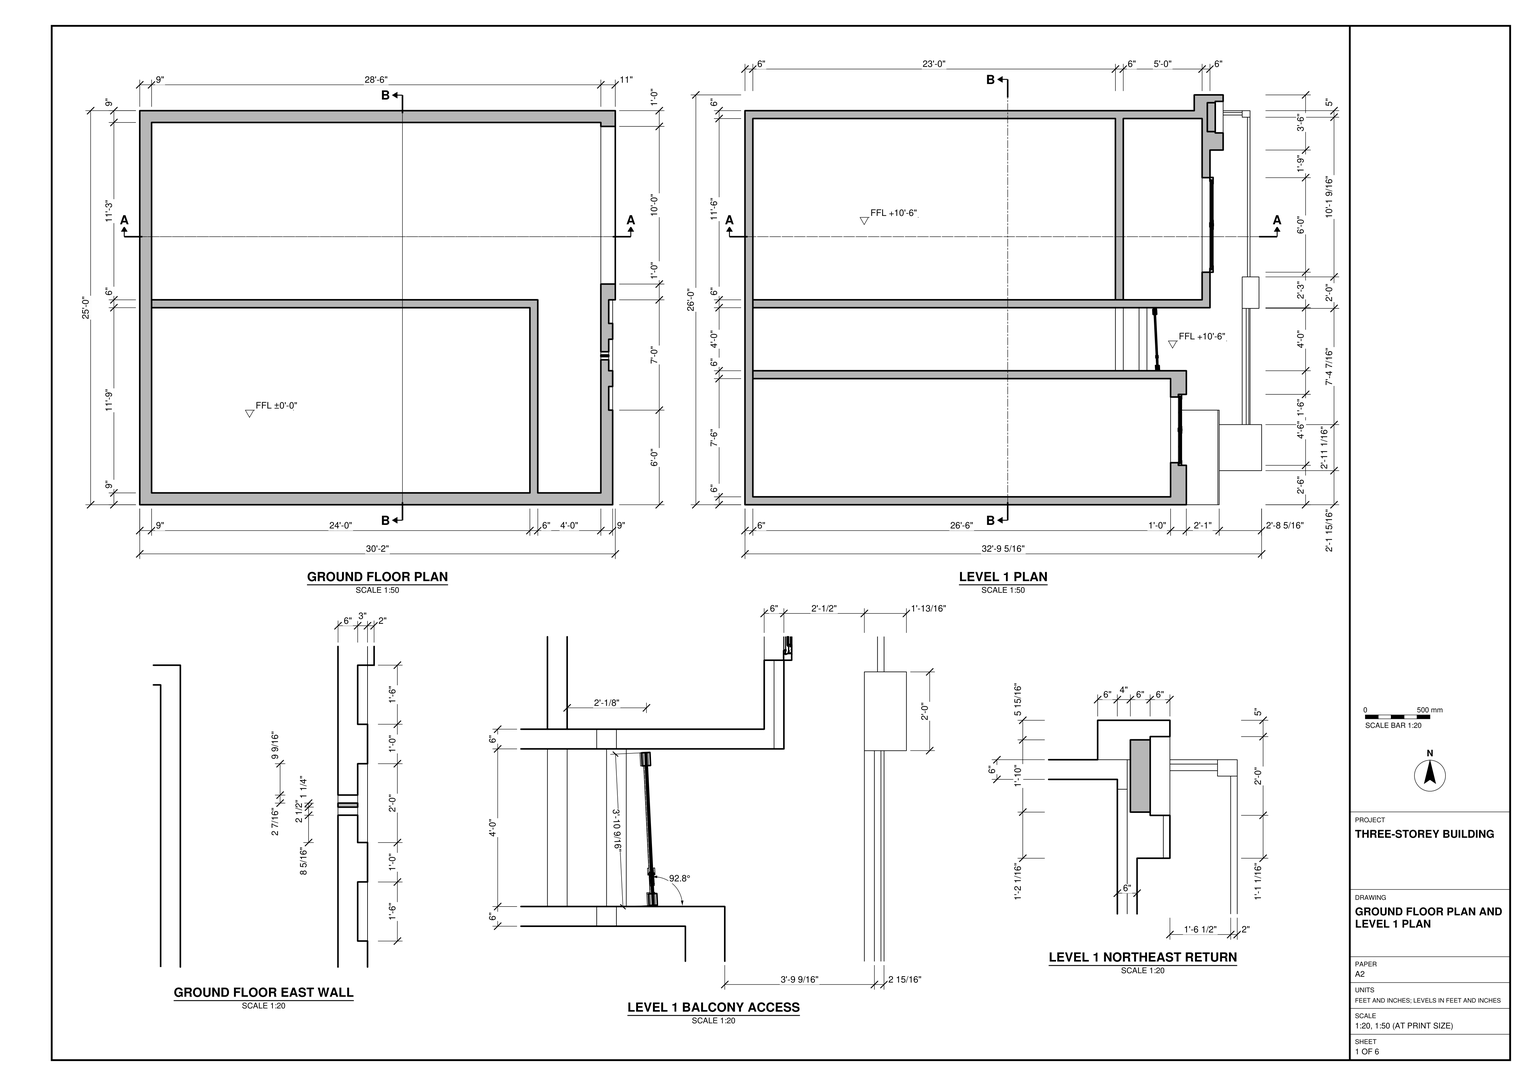
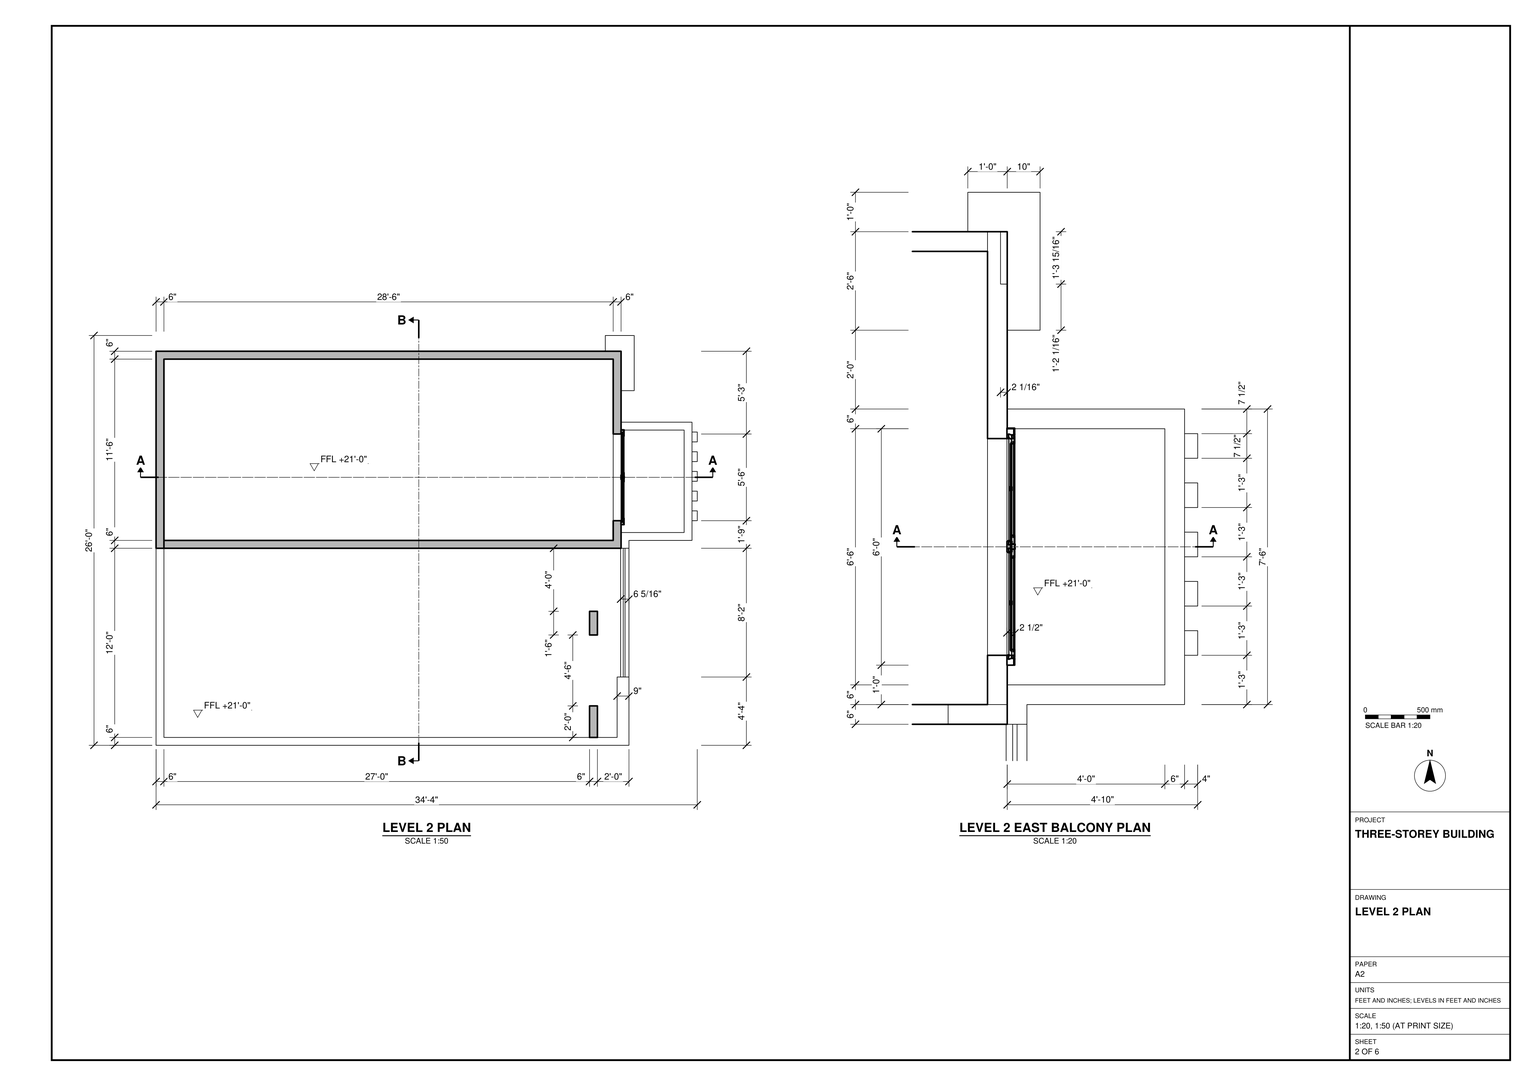
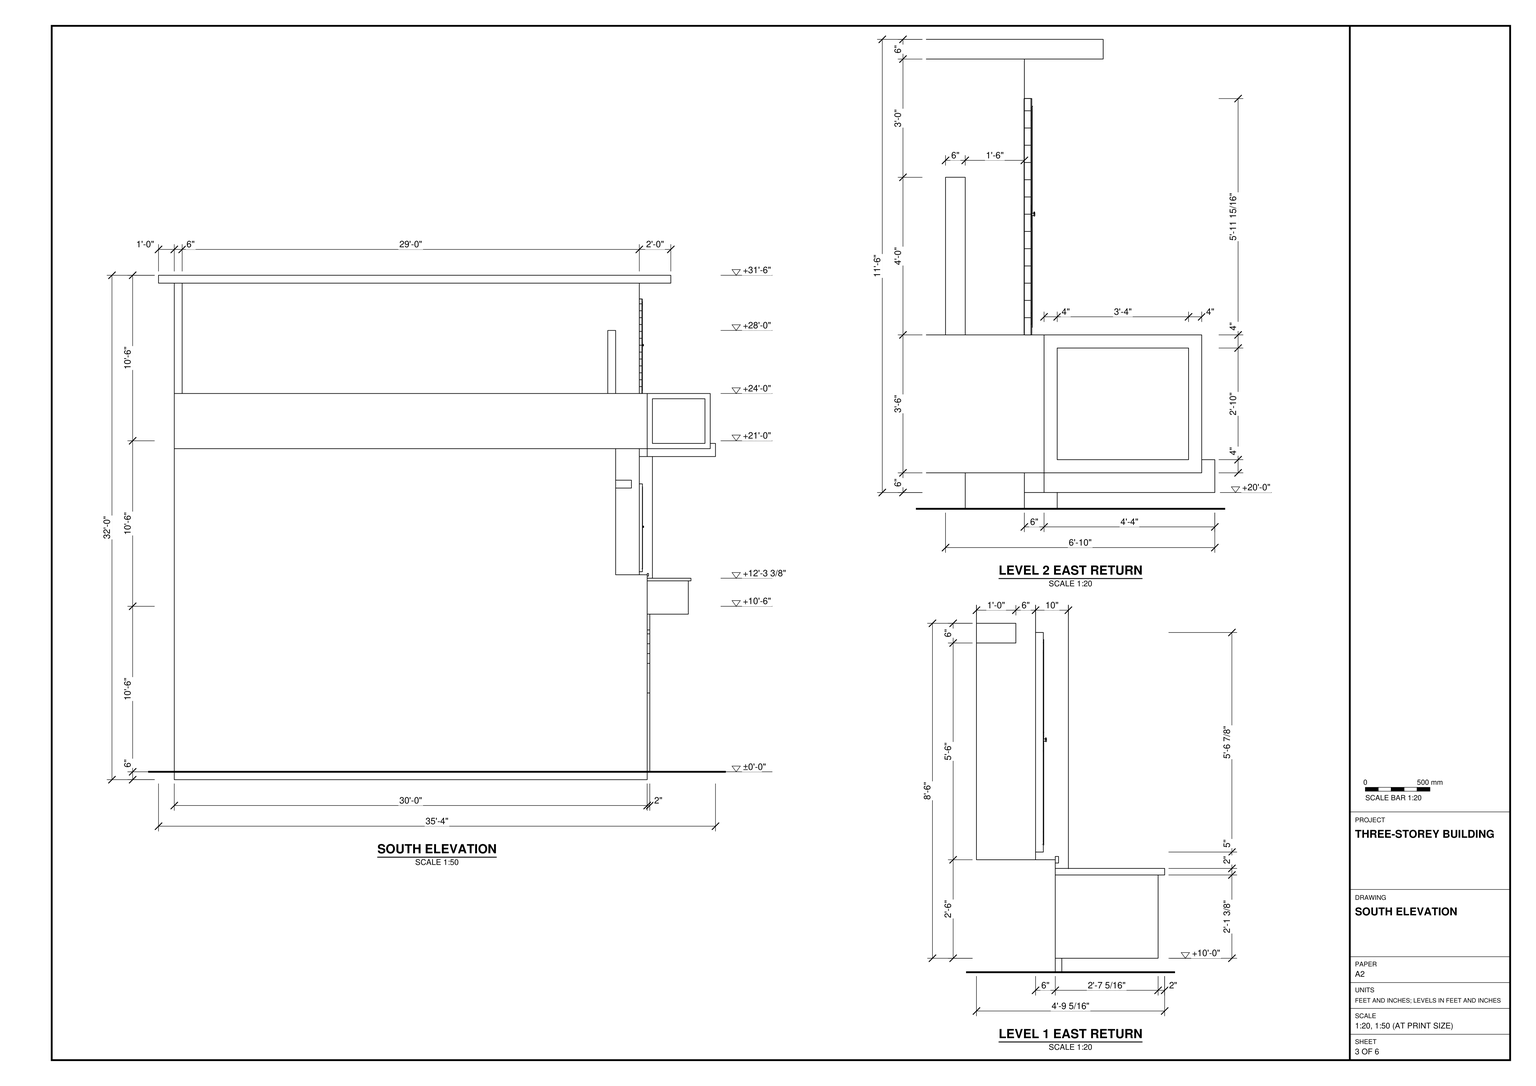
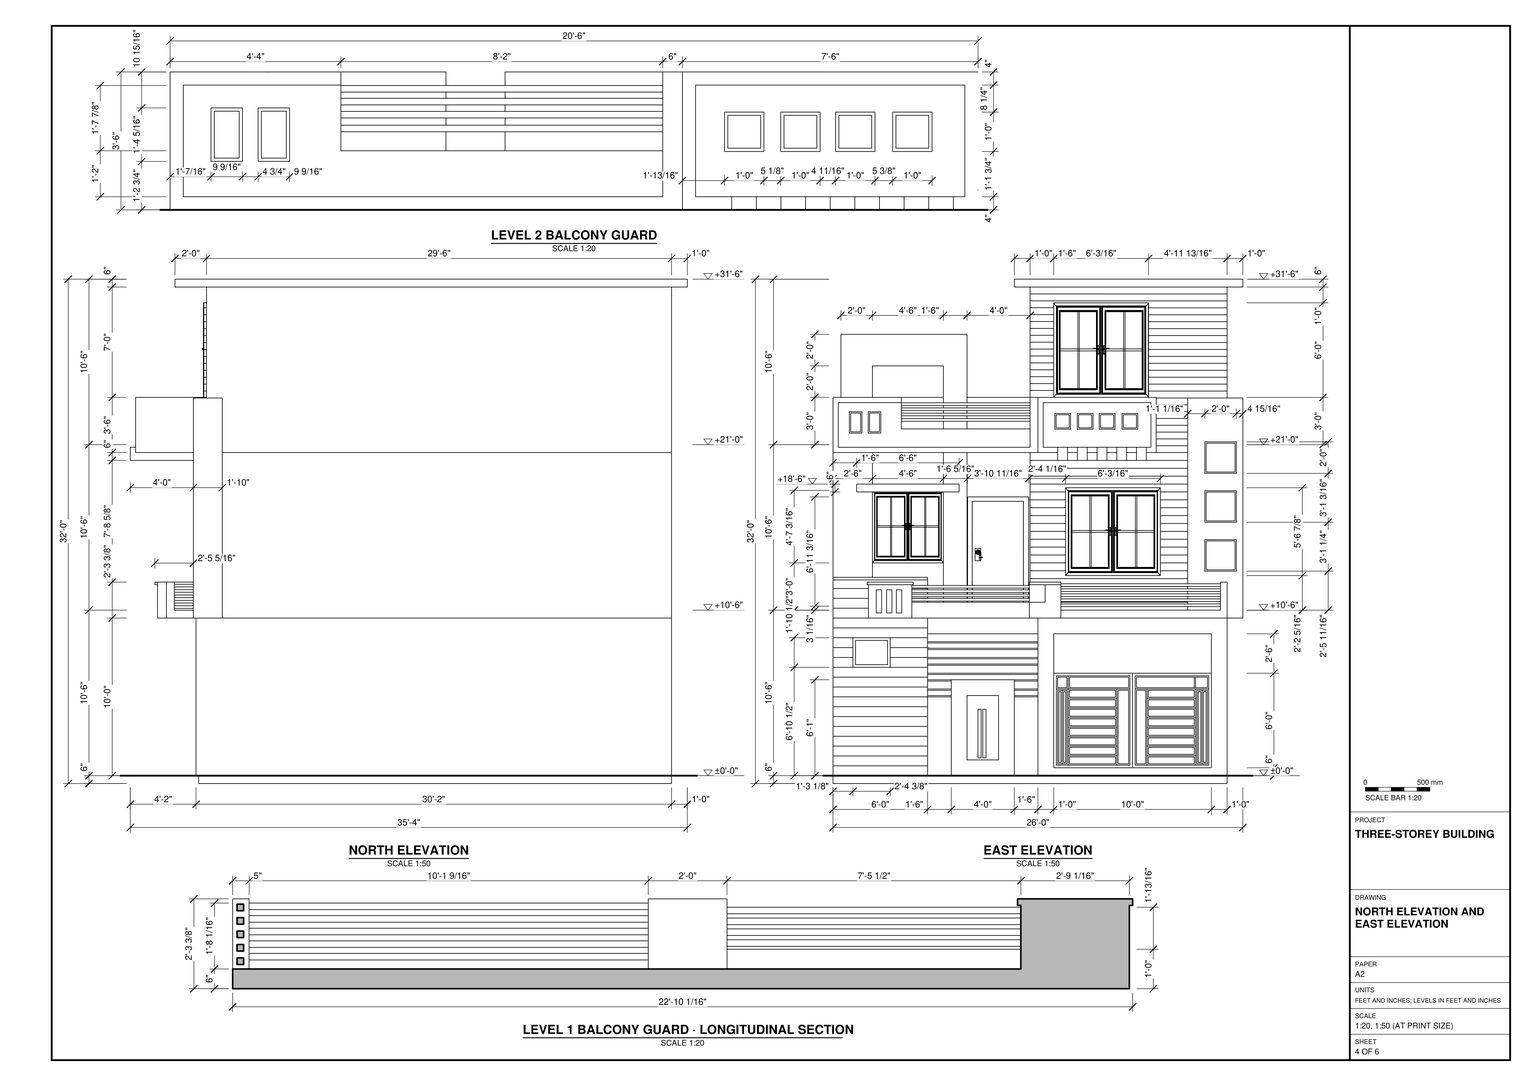
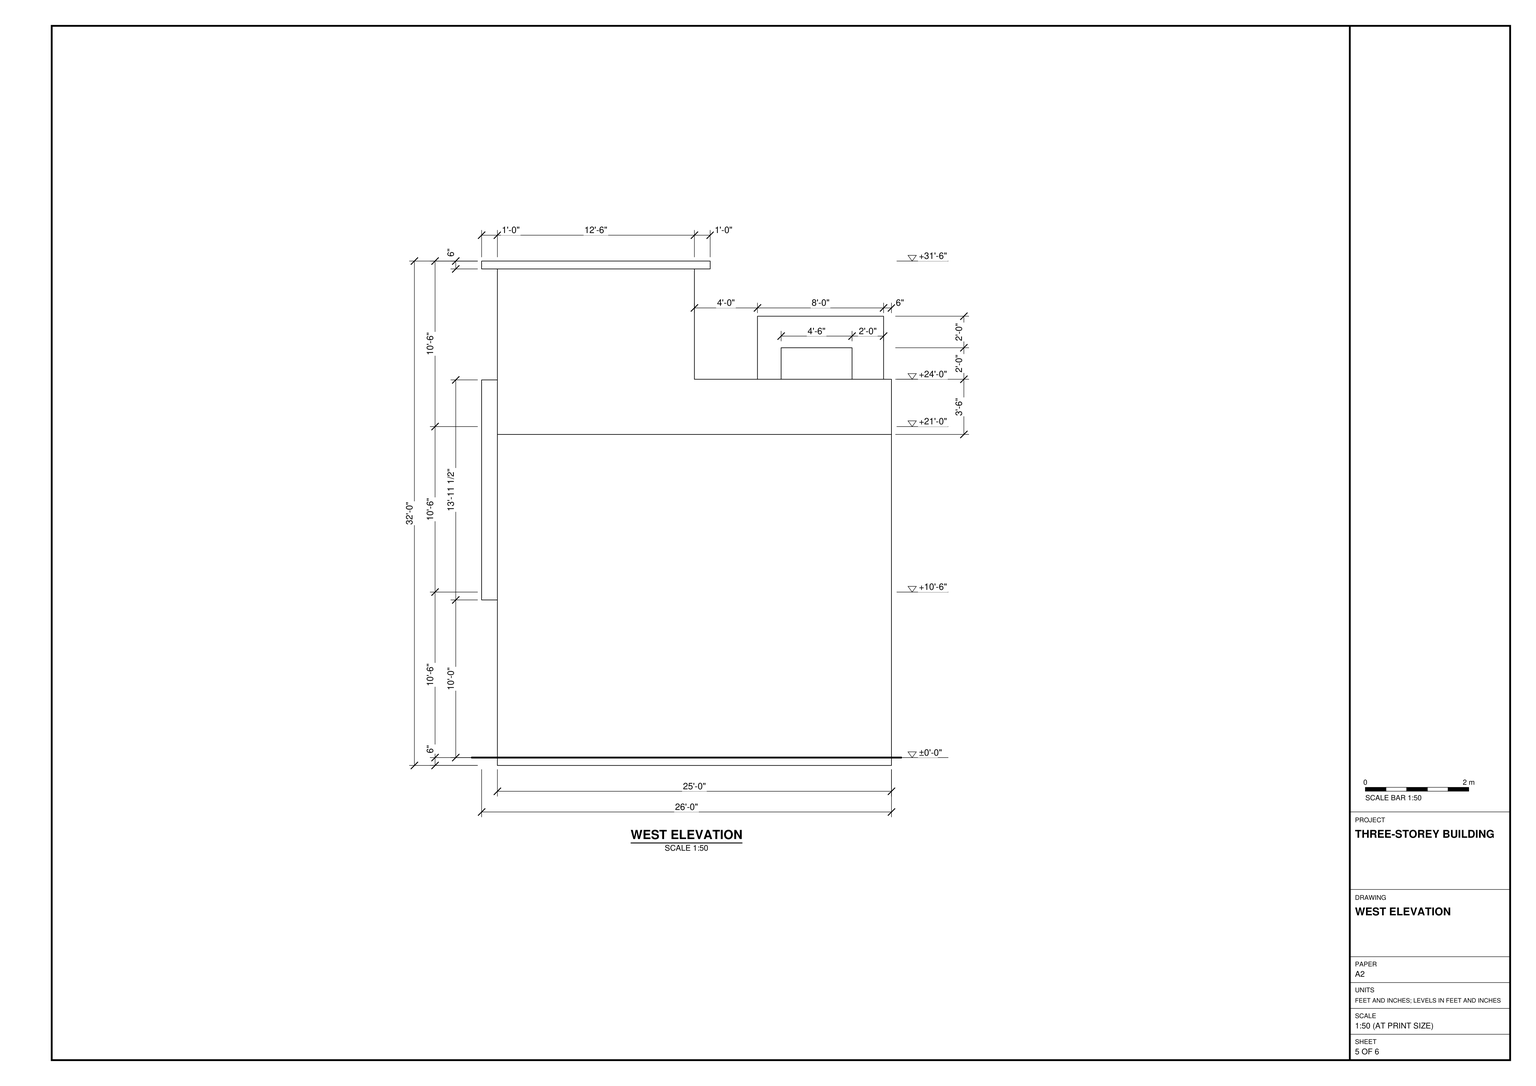
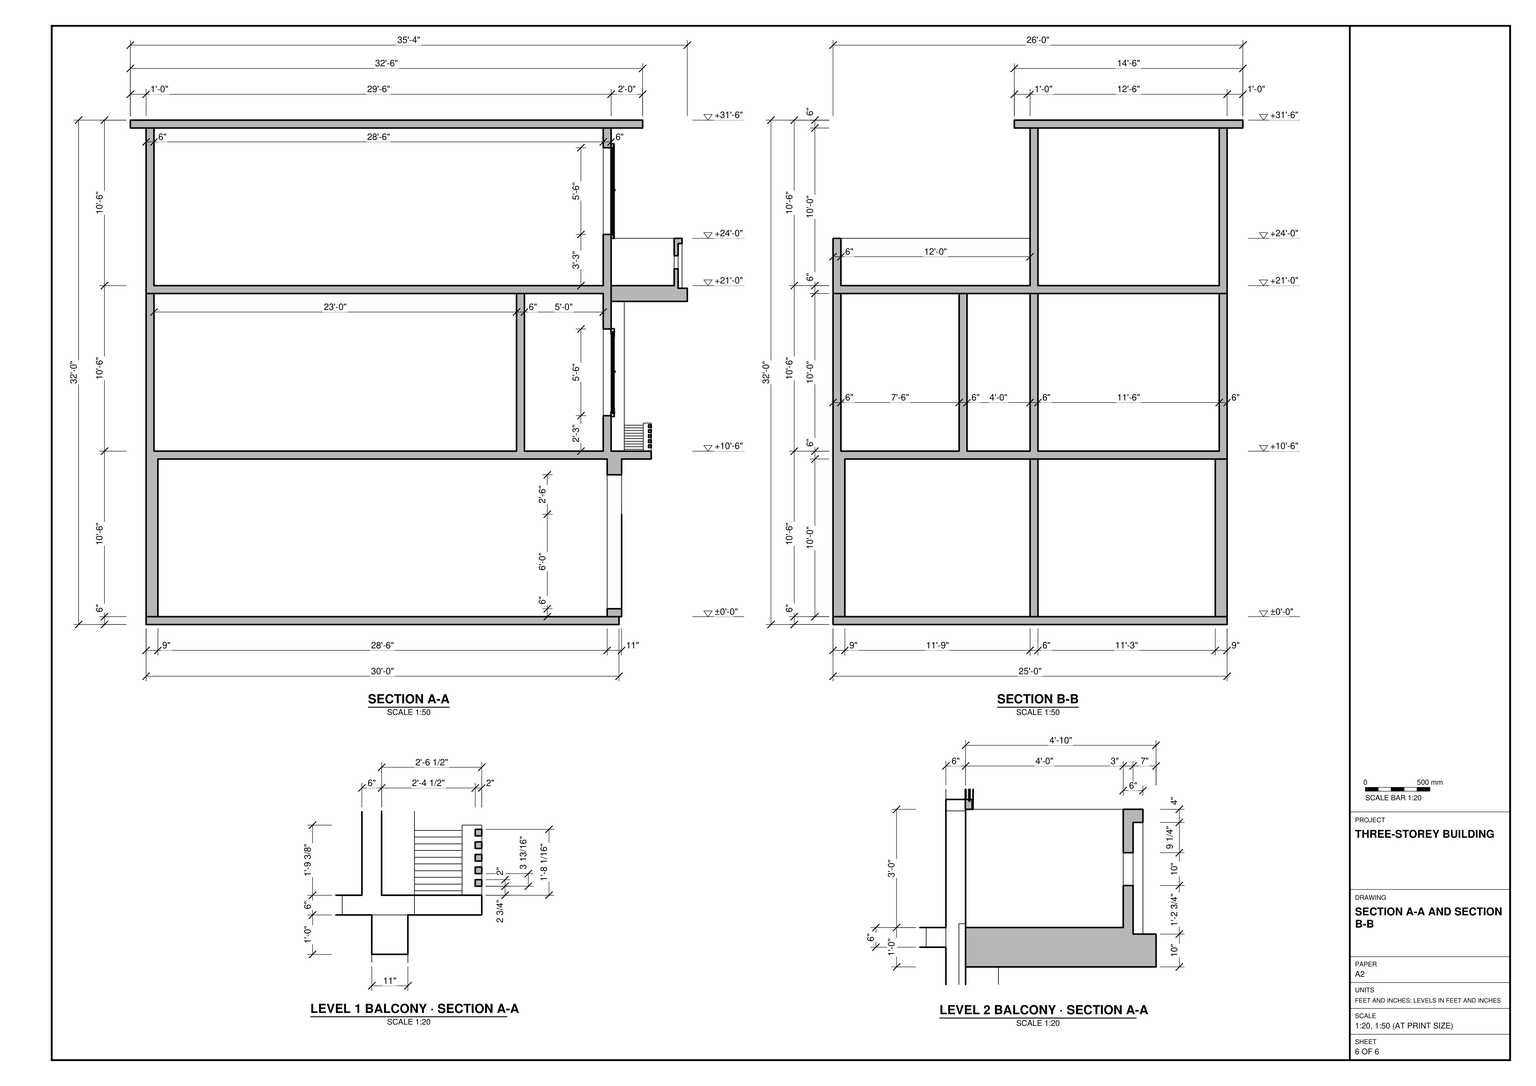
Build the three-storey building in SketchUp from task_files/diagram_01.pdf. Work in feet and inches. The overall model measures 35'-4" east to west, 26'-0" north to south and 32'-0" from the underside of the base slab to the top of the roof. Set the finished floor levels at ±0'-0", +10'-6" and +21'-0".

Follow the wall thicknesses on each plan rather than using one thickness throughout. On the ground floor, model the 9" perimeter walls where indicated and the 6" partition that turns south near the east wall. Form the east wall openings and recesses as drawn. On Level 1, divide the north room to form the narrow east bay and leave the passage between the north and south rooms leading to the balcony. On Level 2, enclose the north room and retain the terrace to its south. Use the enlarged balcony plans and return details to model the access openings, projecting slabs, balcony edges and repeated projections on the upper balcony face. Match the flat roof overhangs to the south elevation.

Include stairs, built-in joinery and main furniture only where shown. Keep walls, slabs, the roof and each furniture or joinery piece in separate groups or components, and use components for repeated parts. Any decor or loose items shown may be represented by suitable library components. Save one SketchUp model as output_files/three_storey_building_with_balconies_and_south_terrace.skp.

# SketchUp Ruby script. Lengths in inches.
U = 1.inch
M = Sketchup.active_model
def pt(a) = Geom::Point3d.new(a.map { |v| v * U })
def face(e, loops, mat)
  f = e.add_face(loops[0].map { |a| pt(a) })
  loops[1..].each { |l| e.add_face(l.map { |a| pt(a) }).erase! }
  f.material = f.back_material = mat if mat
  f
end
# faces: each face lists its corners as indices into pts; further lists are holes
def faces(e, pts, list, mat = nil) = list.each { |f| face(e, (f[0].is_a?(Array) ? f : [f]).map { |l| l.map { |i| pts[i] } }, mat) }
# xy, xz, yz: faces in a plane at the given z, y or x. An outline is a flat list of corners, or four numbers for a rectangle; further outlines are holes
def ring(l) = l.size == 4 ? [[l[0], l[1]], [l[2], l[1]], [l[2], l[3]], [l[0], l[3]]] : l.each_slice(2).to_a
def flat(e, list, mat, &to3) = list.each { |f| face(e, (f[0].is_a?(Array) ? f : [f]).map { |l| ring(l).map { |u, v| to3.(u, v) } }, mat) }
def xy(e, z, list, mat = nil) = flat(e, list, mat) { |x, y| [x, y, z] }
def xz(e, y, list, mat = nil) = flat(e, list, mat) { |x, z| [x, y, z] }
def yz(e, x, list, mat = nil) = flat(e, list, mat) { |y, z| [x, y, z] }
def lines(e, pts, list) = list.each { |a, b| e.add_line(pt(pts[a]), pt(pts[b])) }
# prism: a flat outline (further loops are holes) pulled along v
def prism(e, loops, v, mat = nil)
  f = face(e, loops, mat); d = Geom::Vector3d.new(v.map { |x| x * U })
  f.pushpull(f.normal.samedirection?(d) ? d.length : -d.length)
end
def box(e, o, s, mat = nil) = prism(e, [[o, [o[0] + s[0], o[1], o[2]], [o[0] + s[0], o[1] + s[1], o[2]], [o[0], o[1] + s[1], o[2]]]], [0, 0, s[2]], mat)
def at(x, y, z, deg = 0) = Geom::Transformation.translation(pt([x, y, z])) * Geom::Transformation.rotation(ORIGIN, Z_AXIS, deg.degrees)
def axes(o, x, y, z) = Geom::Transformation.new([*x, 0, *y, 0, *z, 0, *pt(o).to_a, 1])
def part(name) = M.definitions.add(name)
# library, detail: a bought-in or finely detailed component or shape, given as its bounding box
def library(name, o, s) = part(name).tap { |d| box(d.entities, o, s) }
def detail(e, o, s) = box(e.add_group.entities, o, s)
def put(e, d, t, mat = nil) = e.add_instance(d, t).tap { |i| i.material = mat if mat }
def group(e, t, mat = nil) = e.add_group.tap { |g| g.transformation = t; g.material = mat if mat }.entities
root = M.entities
M.materials.add("A08_Garnet_Shadow").color = [102, 0, 0]
M.materials.add("D07_Ochre_Flame").color = [153, 107, 0]
M.materials.add("Denim_03_1K").color = [93, 106, 119]
M.materials.add("Glass_Basic_01").color = [75, 19, 186]
M.materials["Glass_Basic_01"].alpha = 0.25
M.materials.add("Wood_Veneer_15_1K").color = [103, 69, 45]
c1 = library("porta+4",[0.2,-5.42,1.33],[46.55,4.72,83.21])
c2 = library("mesh-163",[-551.08,-704.17,-20.03],[1929.24,1401.85,86.96])
c3 = part("Group11\#1")
put(c3.entities,c2,at(0,0,0))
xy(root,-6,[[12,0,372,300]])
xy(root,0,[[12,0,309,9],[309,0,309,150,21,150,21,156,315,156,315,0],[315,0,372,9],[12,9,21,150],[21,9,309,150],
  [315,9,363,9,363,291,21,291,21,156,315,156],[363,9,363,291,372,291,372,156,369,156,369,138,372,138,372,90,369,90,369,72,372,72,372,9],[369,72,372,90],[369,138,372,156],[12,150,21,156],
  [12,156,21,300],[21,291,372,300]])
xy(root,0,[[372,156,374,291],[372,291,374,300]],"Wood_Veneer_15_1K")
xy(root,6,[[363,168,374,288]],"Wood_Veneer_15_1K")
xy(root,12,[[369,102,372,126]])
xy(root,13.55,[[363,110.32,369,112.77],[363,114,369,116.45]],"D07_Ochre_Flame")
xy(root,50.58,[[363,110.32,369,112.77],[363,114,369,116.45]],"D07_Ochre_Flame")
xy(root,61,[[363,72,369,90],[369,102,372,126],[363,138,369,156]])
xy(root,65,[[363,72,369,90],[363,138,369,156]])
xy(root,66,[[363,72,369,90],[363,138,369,156]])
xy(root,72,[[363,72,369,90],[363,138,369,156]])
xy(root,73,[[363,72,369,72,369,90,372,90,372,138,369,138,369,156,363,156]])
xy(root,77,[[363,72,369,90],[363,90,369,138],[363,138,369,156]])
xy(root,78,[[363,72,369,156]])
xy(root,82.5,[[372,15.15,374,43.52]])
xy(root,84,[[363,72,369,90],[363,90,369,138],[363,138,369,156]])
xy(root,84.5,[[363,17.15,374,41.52]],"Denim_03_1K")
xy(root,85,[[363,72,369,156]])
xy(root,89,[[363,72,369,90],[363,90,369,138],[363,138,369,156]])
xy(root,90,[[363,72,369,90],[363,90,369,156]])
xy(root,96,[[363,72,369,90],[363,90,369,138],[363,138,369,156]])
xy(root,97,[[363,72,369,73],[363,73,369,90],[363,90,369,156]])
xy(root,101,[[363,72,369,90],[363,90,369,138],[363,138,369,156]])
xy(root,102,[[363,72,369,90],[363,90,369,156]])
xy(root,103,[[363,17.15,374,41.52]],"Denim_03_1K")
xy(root,105,[[372,15.15,374,43.52]])
xy(root,108,[[363,72,372,156]])
xy(root,108,[[363,168,374,288]],"Wood_Veneer_15_1K")
xy(root,120,[[21,9,309,150],[315,9,363,291],[372,26.95,372,156,403.3125,156,403.3125,149.46,396.5,149.46,396.5,60,403.3125,60,403.3125,26.95],[21,150,309,156],[21,156,309,291],
  [309,156,315,291],[374,156,374,300,396.5,300,396.5,173.46,403.3125,173.46,403.3125,156],[21,291,309,300],[309,291,315,300],[315,291,363,300]])
xy(root,120,[[354,300,376,312]],"D07_Ochre_Flame")
xy(root,123.88,[[398.5,32.9,403.3125,36.99],[398.5,40.77,403.3125,44.86],[398.5,48.2,403.3125,52.29]])
xy(root,126,[[18,6,336,96],[372,60,390.5,60,390.5,173.46,396.5,173.46,396.5,295,390.5,295,390.5,300,376,300,376,270,366,270,366,150,318,150,318,102,348,102,348,84,342,84,342,72,372,72],[18,102,294,150],[294,102,300,150],[300,102,312,150],
  [312,102,318,150],[18,156,294,294],[300,156,360,294]])
xy(root,127.37,[[376,296.66,390.5,298.66]])
xy(root,128.75,[[394.5,173.46,396.5,295]])
xy(root,129.37,[[376,296.66,390.5,298.66]])
xy(root,130.75,[[394.5,173.46,396.5,295]])
xy(root,131.46,[[376,296.66,390.5,298.66]])
xy(root,132,[[390.5,60,396.5,149.46]])
xy(root,132,[[396.5,149.46,403.3125,161.46]],"D07_Ochre_Flame")
xy(root,132.58,[[394.5,173.46,396.5,295]])
xy(root,132.91,[[393.55,60,395.55,149.46]])
xy(root,133.46,[[376,296.66,390.5,298.66]])
xy(root,134.58,[[394.5,173.46,396.5,295]])
xy(root,134.91,[[393.55,60,395.55,149.46]])
xy(root,135.55,[[376,296.66,390.5,298.66]])
xy(root,136.21,[[393.55,60,395.55,149.46]])
xy(root,136.41,[[394.5,173.46,396.5,295]])
xy(root,137.55,[[376,296.66,390.5,298.66]])
xy(root,138.21,[[393.55,60,395.55,149.46]])
xy(root,138.41,[[394.5,173.46,396.5,295]])
xy(root,139.51,[[393.55,60,395.55,149.46]])
xy(root,139.64,[[376,296.66,390.5,298.66]])
xy(root,140.24,[[394.5,173.46,396.5,295]])
xy(root,141.5,[[398.5,32.9,403.3125,36.99],[398.5,40.77,403.3125,44.86],[398.5,48.2,403.3125,52.29]])
xy(root,141.51,[[393.55,60,395.55,149.46]])
xy(root,141.64,[[376,296.66,390.5,298.66]])
xy(root,142.24,[[394.5,173.46,396.5,295]])
xy(root,142.8125,[[393.55,60,395.55,149.46]])
xy(root,143.73,[[376,296.66,390.5,298.66]])
xy(root,144.08,[[394.5,173.46,396.5,295]])
xy(root,144.8125,[[393.55,60,395.55,149.46]])
xy(root,145.36,[[372,25.95,396,26.95],[396,25.95,396.5,26.95],[396.5,25.95,405.3125,26.95],[403.3125,26.95,405.3125,60],[372,60,396.5,61],
  [396.5,60,405.3125,61]])
xy(root,145.36,[[396.5,149.46,403.3125,161.46]],"D07_Ochre_Flame")
xy(root,145.73,[[376,296.66,390.5,298.66]])
xy(root,146.08,[[394.5,173.46,396.5,295]])
xy(root,147.36,[[372,25.95,405.3125,61],[390.5,149.46,403.3125,173.46],[390.5,295,396.5,300]])
xy(root,149,[[372,0,373,9],[372,9,373,72]])
xy(root,150,[[348,0,372,0,372,72,342,72,342,30,348,30]])
xy(root,151,[[372,0,373,72]])
xy(root,153,[[360,177,366,249]])
xy(root,155.71,[[370,283.04,376,307.04]],"D07_Ochre_Flame")
xy(root,156.71,[[363.96,284.04,370,306.04]])
xy(root,164,[[336,32,342,82]])
xy(root,178.71,[[363.96,284.04,370,306.04]])
xy(root,179.71,[[370,283.04,376,307.04]],"D07_Ochre_Flame")
xy(root,192.9375,[[370,283.04,376,307.04]],"D07_Ochre_Flame")
xy(root,193.9375,[[363.96,284.04,370,306.04]])
xy(root,210,[[312,102,318,150]])
xy(root,214,[[336,32,342,82]])
xy(root,215.9375,[[363.96,284.04,370,306.04]])
xy(root,216,[[348,18,348,30,342,30,342,84,348,84,348,96,360,96,360,18]])
xy(root,216.9375,[[370,283.04,376,307.04]],"D07_Ochre_Flame")
xy(root,219,[[360,177,366,249]])
xy(root,222,[[348,18,360,18,360,96,348,96,348,84,342,84,342,30,348,30]])
xy(root,230.15,[[370,283.04,376,307.04]],"D07_Ochre_Flame")
xy(root,231.15,[[363.96,284.04,370,306.04]])
xy(root,240,[[366,171,424,178.5],[366,186,424,193.5],[366,201,424,208.5],[366,216,424,223.5],[366,231,424,238.5]],"A08_Garnet_Shadow")
xy(root,246,[[12,0,18,294],[18,0,294,6],[294,0,300,6],[300,0,348,6],[348,0,348,30,342,30,342,84,348,84,348,102,318,102,318,150,366,150,366,171,420,171,420,156,372,156,372,0],
  [18,6,336,96],[336,6,348,6,348,30,342,30,342,84,348,84,348,96,336,96],[18,96,294,102],[294,96,300,102],[300,96,348,96,348,102,318,102,318,150,312,150,312,102,300,102],
  [18,102,294,150],[294,102,300,150],[300,102,312,150],[18,150,294,156],[294,150,300,156],
  [300,150,318,156],[318,150,348,156],[348,150,366,156],[18,156,294,294],[294,156,300,300],
  [300,156,360,294],[366,178.5,420,186],[366,193.5,420,201],[366,208.5,420,216],[366,223.5,420,231],
  [366,238.5,420,246],[12,294,294,300],[300,294,360,300]])
xy(root,250,[[369,4,372,6],[369,6,372,30],[369,30,372,84],[369,84,372,150],[376,156,416,159],
  [417,160,420,171],[417,178.5,420,186],[417,193.5,420,201],[417,208.5,420,216],[417,223.5,420,231],
  [417,238.5,420,242]])
xy(root,250,[[417,171,424,178.5],[417,186,424,193.5],[417,201,424,208.5],[417,216,424,223.5],[417,231,424,238.5]],"A08_Garnet_Shadow")
xy(root,252,[[18,6,342,6,342,30,348,30,348,6,363,6,363,52,366,52,366,150,18,150],[342,6,348,30],[18,156,360,294],[366,162,414,240]])
xy(root,253.15,[[363.96,284.04,370,306.04]])
xy(root,254.15,[[370,283.04,376,307.04]],"D07_Ochre_Flame")
xy(root,260.76,[[369,12.45,370,22.03],[369,26.8,370,36.38]])
xy(root,261.76,[[369,13.45,370,21.03],[369,27.8,370,35.38]])
xy(root,264,[[366,52,369,150]])
xy(root,264.78,[[414,169.82,417,179.82],[414,186.93,417,196.93],[414,203.64,417,213.64],[414,221.01,417,231.01]])
xy(root,269.79,[[365.66,52,367.66,150]])
xy(root,271.79,[[365.66,52,367.66,150]])
xy(root,273.99,[[365.66,52,367.66,150]])
xy(root,274.78,[[414,169.82,417,179.82],[414,186.93,417,196.93],[414,203.64,417,213.64],[414,221.01,417,231.01]])
xy(root,275.99,[[365.66,52,367.66,150]])
xy(root,276.05,[[369,13.45,370,21.03],[369,27.8,370,35.38]])
xy(root,277.05,[[369,12.45,370,22.03],[369,26.8,370,36.38]])
xy(root,277.97,[[365.66,52,367.66,150]])
xy(root,279.97,[[365.66,52,367.66,150]])
xy(root,281.87,[[365.66,52,367.66,150]])
xy(root,283.87,[[365.66,52,367.66,150]])
xy(root,284,[[369,4,372,52],[376,156,416,159],[417,160,420,242]])
xy(root,287.51,[[366,270,376,270,376,312,354,312,354,300,366,300]],"D07_Ochre_Flame")
xy(root,288,[[12,0,372,0,372,52,363,52,363,6,18,6,18,150,12,150],[366,150,372,150,372,156,420,156,420,246,366,246,366,240,414,240,414,162,366,162],[366,168,368,240]])
xy(root,291,[[360,171,368,237]])
xy(root,312,[[342,30,348,84]])
xy(root,336,[[342,6,348,102]],"D07_Ochre_Flame")
xy(root,357,[[360,171,368,237]])
xy(root,360,[[366,168,368,240]])
xy(root,372,[[0,138,12,300],[12,138,18,150],[18,138,18,150,366,150,366,300,18,300,18,312,390,312,390,138],[12,150,18,300],[18,150,318,156],
  [318,150,366,156],[18,156,360,294],[360,156,366,162],[360,162,366,294],[18,294,366,300],
  [0,300,18,312]])
xy(root,378,[[0,138,390,312]])
xz(root,0,[[12,-6,372,0],[12,0,372,0,372,150,348,150,348,246,12,246],[372,149,373,151],[12,246,372,288]])
xz(root,4,[[369,250,372,284]])
xz(root,6,[[18,126,336,246],[18,252,342,288],[342,252,348,288],[348,252,363,288]])
xz(root,6,[[342,288,348,336]],"D07_Ochre_Flame")
xz(root,9,[[21,0,309,120],[315,0,363,120]])
xz(root,12.45,[[369,260.76,370,277.05]])
xz(root,13.45,[[369,261.76,370,276.05]])
xz(root,15.15,[[372,82.5,374,90],[372,90,374,97.5],[372,97.5,374,105]])
xz(root,17.15,[[363,84.5,374,90],[363,90,374,97.5],[363,97.5,374,103]],"Denim_03_1K")
xz(root,18,[[348,216,360,222]])
xz(root,21.03,[[369,261.76,370,276.05]])
xz(root,22.03,[[369,260.76,370,277.05]])
xz(root,25.95,[[372,145.36,405.3125,147.36]])
xz(root,26.8,[[369,260.76,370,277.05]])
xz(root,26.95,[[372,120,403.3125,145.36]])
xz(root,27.8,[[369,261.76,370,276.05]])
xz(root,30,[[342,252,348,312]])
xz(root,30,[[342,150,348,216],[342,222,348,246]],"D07_Ochre_Flame")
xz(root,32,[[336,164,342,214]])
xz(root,32.9,[[398.5,123.88,403.3125,141.5]])
xz(root,35.38,[[369,261.76,370,276.05]])
xz(root,36.38,[[369,260.76,370,277.05]])
xz(root,36.99,[[398.5,123.88,403.3125,141.5]])
xz(root,40.77,[[398.5,123.88,403.3125,141.5]])
xz(root,41.52,[[363,84.5,374,90],[363,90,374,97.5],[363,97.5,374,103]],"Denim_03_1K")
xz(root,43.52,[[372,82.5,374,90],[372,90,374,97.5],[372,97.5,374,105]])
xz(root,44.86,[[398.5,123.88,403.3125,141.5]])
xz(root,48.2,[[398.5,123.88,403.3125,141.5]])
xz(root,52,[[[363,252,363,288,372,288,372,284,369,284,369,264,366,264,366,252],[365.66,281.87,367.66,283.87],[365.66,277.97,367.66,279.97],[365.66,273.99,367.66,275.99],[365.66,269.79,367.66,271.79]]])
xz(root,52.29,[[398.5,123.88,403.3125,141.5]])
xz(root,60,[[[372,126,372,145.36,403.3125,145.36,403.3125,126,396.5,126,396.5,132,390.5,132,390.5,126],[393.55,142.8125,395.55,144.8125],[393.55,139.51,395.55,141.51],[393.55,136.21,395.55,138.21],[393.55,132.91,395.55,134.91]]])
xz(root,60,[[396.5,120,403.3125,126]],"D07_Ochre_Flame")
xz(root,61,[[372,145.36,405.3125,147.36]])
xz(root,72,[[369,0,372,7.5],[369,7.5,372,15],[369,15,372,22.5],[369,22.5,372,30],[369,30,372,37.5],
  [369,37.5,372,45],[369,45,372,52.5],[369,52.5,372,60],[369,60,369,61,363,61,363,65,369,65,369,66,363,66,363,67.5,372,67.5,372,60],[363,67.5,363,72,369,72,369,73,363,73,363,75,372,75,372,67.5],
  [363,75,363,77,369,77,369,78,363,78,363,82.5,372,82.5,372,75],[363,82.5,363,84,369,84,369,85,363,85,363,89,369,89,369,90,372,90,372,82.5],[363,90,363,96,369,96,369,97,363,97,363,97.5,372,97.5,372,90],[363,97.5,363,101,369,101,369,102,363,102,363,105,372,105,372,97.5],[363,105,372,108],
  [342,126,342,150,372,150,372,151,373,151,373,149,372,149,372,126]])
xz(root,82,[[336,164,342,214]])
xz(root,84,[[342,126,348,216],[342,222,348,246],[342,252,348,312]],"D07_Ochre_Flame")
xz(root,90,[[369,0,372,0,372,73,369,73,369,72,363,72,363,66,369,66,369,65,363,65,363,61,369,61]])
xz(root,96,[[18,126,336,246],[348,216,360,222]])
xz(root,102,[[369,12,372,61],[18,126,294,246],[294,126,300,246],[300,126,312,246],[312,126,318,210],
  [318,126,348,246],[342,252,348,336]])
xz(root,110.32,[[363,13.55,369,50.58]],"D07_Ochre_Flame")
xz(root,112.77,[[363,13.55,369,50.58]],"D07_Ochre_Flame")
xz(root,114,[[363,13.55,369,50.58]],"D07_Ochre_Flame")
xz(root,116.45,[[363,13.55,369,50.58]],"D07_Ochre_Flame")
xz(root,126,[[369,12,372,61]])
xz(root,138,[[369,0,369,61,363,61,363,65,369,65,369,66,363,66,363,72,369,72,369,73,372,73,372,0],[0,372,390,378]])
xz(root,149.46,[[396.5,120,403.3125,132],[[390.5,132,396.5,132,396.5,145.36,403.3125,145.36,403.3125,147.36,390.5,147.36],[393.55,132.91,395.55,134.91],[393.55,136.21,395.55,138.21],[393.55,139.51,395.55,141.51],[393.55,142.8125,395.55,144.8125]]])
xz(root,149.46,[[396.5,132,403.3125,145.36]],"Glass_Basic_01")
xz(root,150,[[21,0,309,120],[18,126,294,246],[294,126,300,246],[300,126,312,246],[312,126,318,210],
  [318,126,366,246],[18,252,366,252,366,269.79,365.66,269.79,365.66,271.79,366,271.79,366,273.99,365.66,273.99,365.66,275.99,366,275.99,366,277.97,365.66,277.97,365.66,279.97,366,279.97,366,281.87,365.66,281.87,365.66,283.87,366,283.87,366,372,18,372],[366,252,369,264],[365.66,269.79,366,271.79],[366,269.79,367.66,271.79],
  [365.66,273.99,366,275.99],[366,273.99,367.66,275.99],[365.66,277.97,366,279.97],[366,277.97,367.66,279.97],[365.66,281.87,366,283.87],
  [366,281.87,367.66,283.87],[12,288,18,372]])
xz(root,156,[[21,0,315,120],[18,126,294,246],[294,126,300,246],[300,126,360,246],[[372,246,420,288],[376,250,416,284]],
  [18,252,318,372],[318,252,360,372]])
xz(root,156,[[369,0,374,60],[369,60,374,60,374,108,363,108,363,102,369,102,369,101,363,101,363,97,369,97,369,96,363,96,363,90,369,90,369,89,363,89,363,85,369,85,369,84,363,84,363,78,369,78,369,77,363,77,363,73,369,73,369,72,363,72,363,66,369,66,369,65,363,65,363,61,369,61],[372,108,374,120]],"Wood_Veneer_15_1K")
xz(root,159,[[376,250,416,284]])
xz(root,160,[[417,250,420,284]])
xz(root,161.46,[[396.5,132,403.3125,145.36]],"D07_Ochre_Flame")
xz(root,162,[[366,252,414,288]])
xz(root,168,[[366,288,368,293.25],[366,293.25,368,298.5],[366,298.5,368,303.75],[366,303.75,368,309],[366,309,368,314.25],
  [366,314.25,368,319.5],[366,319.5,368,324.75],[366,324.75,368,330],[366,330,368,335.25],[366,335.25,368,340.5],
  [366,340.5,368,345.75],[366,345.75,368,351],[366,351,368,356.25],[366,356.25,368,360]])
xz(root,168,[[363,6,374,108]],"Wood_Veneer_15_1K")
xz(root,169.82,[[414,264.78,417,274.78]])
xz(root,171,[[366,240,372,246],[360,291,368,357]])
xz(root,171,[[372,240,424,240,424,250,420,250,420,246,372,246]],"A08_Garnet_Shadow")
xz(root,173.46,[[[396.5,120,396.5,126,390.5,126,390.5,147.36,403.3125,147.36,403.3125,120],[394.5,144.08,396.5,146.08],[394.5,140.24,396.5,142.24],[394.5,136.41,396.5,138.41],[394.5,132.58,396.5,134.58],[394.5,128.75,396.5,130.75]]])
xz(root,177,[[360,153,366,219]])
xz(root,178.5,[[366,240,372,246],[372,240,372,246,420,246,420,250,424,250,424,240]],"A08_Garnet_Shadow")
xz(root,179.82,[[414,264.78,417,274.78]])
xz(root,186,[[366,240,372,246]])
xz(root,186,[[372,240,424,240,424,250,420,250,420,246,372,246]],"A08_Garnet_Shadow")
xz(root,186.93,[[414,264.78,417,274.78]])
xz(root,193.5,[[366,240,372,246],[372,240,372,246,420,246,420,250,424,250,424,240]],"A08_Garnet_Shadow")
xz(root,196.93,[[414,264.78,417,274.78]])
xz(root,201,[[366,240,372,246]])
xz(root,201,[[372,240,424,240,424,250,420,250,420,246,372,246]],"A08_Garnet_Shadow")
xz(root,203.64,[[414,264.78,417,274.78]])
xz(root,208.5,[[366,240,372,246],[372,240,372,246,420,246,420,250,424,250,424,240]],"A08_Garnet_Shadow")
xz(root,213.64,[[414,264.78,417,274.78]])
xz(root,216,[[366,240,372,246]])
xz(root,216,[[372,240,424,240,424,250,420,250,420,246,372,246]],"A08_Garnet_Shadow")
xz(root,221.01,[[414,264.78,417,274.78]])
xz(root,223.5,[[366,240,372,246],[372,240,372,246,420,246,420,250,424,250,424,240]],"A08_Garnet_Shadow")
xz(root,231,[[366,240,372,246]])
xz(root,231,[[372,240,424,240,424,250,420,250,420,246,372,246]],"A08_Garnet_Shadow")
xz(root,231.01,[[414,264.78,417,274.78]])
xz(root,237,[[360,291,368,357]])
xz(root,238.5,[[366,240,372,246],[372,240,372,246,420,246,420,250,424,250,424,240]],"A08_Garnet_Shadow")
xz(root,240,[[366,252,414,288],[366,288,368,292.79],[366,292.79,368,298.08],[366,298.08,368,303.36],[366,303.36,368,308.64],
  [366,308.64,368,313.92],[366,313.92,368,319.2],[366,319.2,368,324.48],[366,324.48,368,329.76],[366,329.76,368,335.04],
  [366,335.04,368,340.32],[366,340.32,368,345.6],[366,345.6,368,350.88],[366,350.88,368,356.16],[366,356.16,368,360]])
xz(root,242,[[417,250,420,284]])
xz(root,246,[[366,246,420,288]])
xz(root,249,[[360,153,366,219]])
xz(root,270,[[366,126,376,287.51]],"D07_Ochre_Flame")
xz(root,283.04,[[370,155.71,376,179.71],[370,192.9375,376,216.9375],[370,230.15,376,254.15]],"D07_Ochre_Flame")
xz(root,284.04,[[363.96,156.71,370,178.71],[363.96,193.9375,370,215.9375],[363.96,231.15,370,253.15]])
xz(root,288,[[363,6,374,108]],"Wood_Veneer_15_1K")
xz(root,291,[[21,0,363,120]])
xz(root,294,[[18,126,294,246],[300,126,360,246],[18,252,360,372]])
xz(root,295,[[390.5,126,396.5,126,396.5,128.75,394.5,128.75,394.5,130.75,396.5,130.75,396.5,132.58,394.5,132.58,394.5,134.58,396.5,134.58,396.5,136.41,394.5,136.41,394.5,138.41,396.5,138.41,396.5,140.24,394.5,140.24,394.5,142.24,396.5,142.24,396.5,144.08,394.5,144.08,394.5,146.08,396.5,146.08,396.5,147.36,390.5,147.36]])
xz(root,296.66,[[376,127.37,390.5,129.37],[376,131.46,390.5,133.46],[376,135.55,390.5,137.55],[376,139.64,390.5,141.64],[376,143.73,390.5,145.73]])
xz(root,298.66,[[376,127.37,390.5,129.37],[376,131.46,390.5,133.46],[376,135.55,390.5,137.55],[376,139.64,390.5,141.64],[376,143.73,390.5,145.73]])
xz(root,300,[[12,-6,372,0],[12,0,374,120],[12,120,354,246],[376,120,376,126,390.5,126,390.5,147.36,396.5,147.36,396.5,120],[12,246,12,372,366,372,366,287.51,354,287.51,354,246],
  [354,246,360,287.51]])
xz(root,306.04,[[363.96,156.71,370,178.71],[363.96,193.9375,370,215.9375],[363.96,231.15,370,253.15]])
xz(root,307.04,[[370,155.71,376,179.71],[370,192.9375,376,216.9375],[370,230.15,376,254.15]],"D07_Ochre_Flame")
xz(root,312,[[0,372,390,378]])
xz(root,312,[[354,120,376,287.51]],"D07_Ochre_Flame")
yz(root,0,[[138,372,312,378]])
yz(root,12,[[0,-6,300,0],[0,0,300,246],[0,246,0,288,150,288,150,372,300,372,300,246]])
yz(root,18,[[6,126,96,246],[96,126,102,246],[102,126,150,246],[150,126,156,246],[156,126,294,246],
  [6,252,150,288],[150,252,156,372],[156,252,294,372]])
yz(root,21,[[9,0,150,120],[150,0,156,120],[156,0,291,120]])
yz(root,294,[[156,126,294,246]])
yz(root,300,[[156,126,294,246]])
yz(root,309,[[9,0,150,120]])
yz(root,312,[[102,210,150,246]])
yz(root,315,[[9,0,156,120]])
yz(root,318,[[102,210,150,246]])
yz(root,336,[[[6,126,96,246],[32,164,82,214]]])
yz(root,342,[[[30,162,84,216],[32,164,82,214]],[30,222,84,246]])
yz(root,342,[[72,126,84,126,84,162,30,162,30,150,72,150],[6,252,6,336,102,336,102,252,84,252,84,312,30,312,30,252]],"D07_Ochre_Flame")
yz(root,348,[[84,126,102,126,102,246,84,246,84,222,96,222,96,216,84,216],[0,150,30,150,30,216,18,216,18,222,30,222,30,246,0,246],[6,252,30,252,30,312,84,312,84,252,102,252,102,336,6,336]],"D07_Ochre_Flame")
yz(root,354,[[300,120,312,287.51]],"D07_Ochre_Flame")
yz(root,360,[[[156,126,294,246],[177,153,249,219]],[18,216,96,222],[156,252,162,372],[[162,252,294,372],[171,291,237,357]]])
yz(root,363,[[[9,0,291,120],[168,6,288,108],[72,78,156,84],[72,90,156,96],[72,102,156,108],[17.15,84.5,41.52,103],[72,73,156,77],[72,85,156,89],[72,97,156,101],[72,66,90,72],[138,66,156,72],[110.32,13.55,112.77,50.58],[114,13.55,116.45,50.58],[138,61,156,65],[72,61,90,65]],[6,252,52,288]])
yz(root,363.96,[[284.04,156.71,306.04,178.71],[284.04,193.9375,306.04,215.9375],[284.04,231.15,306.04,253.15]])
yz(root,365.66,[[52,269.79,150,271.79],[52,273.99,150,275.99],[52,277.97,150,279.97],[52,281.87,150,283.87]])
yz(root,366,[[150,240,171,246],[171,240,178.5,240,178.5,246,186,246,186,240,193.5,240,193.5,246,201,246,201,240,208.5,240,208.5,246,216,246,216,240,223.5,240,223.5,246,231,246,231,240,238.5,240,238.5,246,246,246,246,288,240,288,240,252,162,252,162,288,150,288,150,246,171,246],[178.5,240,186,246],[193.5,240,201,246],[208.5,240,216,246],
  [223.5,240,231,246],[52,252,150,264],[162,252,240,288]])
yz(root,366,[[150,126,270,132],[150,132,270,138],[150,138,270,144],[150,144,270,150],[150,150,270,150,270,156,249,156,249,153,177,153,177,156,150,156],
  [150,156,177,162],[249,156,270,162],[150,162,177,168],[249,162,270,168],[150,168,177,174],
  [249,168,270,174],[150,174,177,180],[249,174,270,180],[150,180,177,186],[249,180,270,186],
  [150,186,177,192],[249,186,270,192],[150,192,177,198],[249,192,270,198],[150,198,177,204],
  [249,198,270,204],[150,204,177,210],[249,204,270,210],[150,210,177,216],[249,210,270,216],
  [150,216,177,216,177,219,249,219,249,216,270,216,270,222,150,222],[150,222,270,228],[150,228,270,234],[150,234,270,240],[238.5,240,270,246],
  [246,246,270,251.1875],[246,251.1875,270,256.38],[246,256.38,270,261.57],[246,261.57,270,266.76],[246,266.76,270,271.95],
  [246,271.95,270,277.14],[246,277.14,270,282.33],[246,282.33,270,287.51],[246,287.51,300,287.51,300,292.79,240,292.79,240,288,246,288],[150,288,168,293.25],
  [240,292.79,300,298.08],[150,293.25,168,298.5],[240,298.08,300,303.36],[150,298.5,168,303.75],[240,303.36,300,308.64],
  [150,303.75,168,309],[240,308.64,300,313.92],[150,309,168,314.25],[240,313.92,300,319.2],[150,314.25,168,319.5],
  [240,319.2,300,324.48],[150,319.5,168,324.75],[240,324.48,300,329.76],[150,324.75,168,330],[240,329.76,300,335.04],
  [150,330,168,335.25],[240,335.04,300,340.32],[150,335.25,168,340.5],[240,340.32,300,345.6],[150,340.5,168,345.75],
  [240,345.6,300,350.88],[150,345.75,168,351],[240,350.88,300,356.16],[150,351,168,356.25],[240,356.16,300,356.16,300,361.4375,168,361.4375,168,361.5,150,361.5,150,356.25,168,356.25,168,360,240,360],
  [168,361.4375,300,361.4375,300,366.72,246,366.72,168,366.75,150,366.75,150,361.5,168,361.5],[246,366.72,300,366.72,300,372,150,372,150,366.75,168,366.75]],"Denim_03_1K")
yz(root,367.66,[[52,269.79,150,271.79],[52,273.99,150,275.99],[52,277.97,150,279.97],[52,281.87,150,283.87]])
yz(root,368,[[[168,288,240,360],[171,291,237,357]]])
yz(root,369,[[72,60,90,61],[138,60,156,61],[72,65,90,66],[138,65,156,66],[72,72,90,73],
  [138,72,156,73],[72,77,156,78],[72,84,156,85],[72,89,156,90],[72,96,156,97],
  [72,101,156,102],[[4,250,150,250,150,264,52,264,52,284,4,284],[26.8,260.76,36.38,277.05],[12.45,260.76,22.03,277.05]],[13.45,261.76,21.03,276.05],[27.8,261.76,35.38,276.05]])
yz(root,369,[[72,0,90,60],[138,0,156,60],[[102,12,126,61],[110.32,13.55,112.77,50.58],[114,13.55,116.45,50.58]]],"D07_Ochre_Flame")
yz(root,370,[[[283.04,155.71,307.04,179.71],[284.04,156.71,306.04,178.71]],[[283.04,192.9375,307.04,216.9375],[284.04,193.9375,306.04,215.9375]],[[283.04,230.15,307.04,254.15],[284.04,231.15,306.04,253.15]],[[12.45,260.76,22.03,277.05],[13.45,261.76,21.03,276.05]],[[26.8,260.76,36.38,277.05],[27.8,261.76,35.38,276.05]]])
yz(root,370,[[284.04,156.71,306.04,178.71],[284.04,193.9375,306.04,215.9375],[284.04,231.15,306.04,253.15]],"Glass_Basic_01")
yz(root,372,[[0,-6,300,0],[[90,0,138,73],[102,12,126,61]],[72,108,156,120],[0,150,72,151],[0,246,156,246,156,288,150,288,150,250,4,250,4,284,52,284,52,288,0,288]])
yz(root,372,[[0,0,72,7.5],[0,7.5,72,15],[0,15,72,22.5],[0,22.5,72,30],[0,30,72,37.5],
  [0,37.5,72,45],[0,45,72,52.5],[0,52.5,72,60],[0,60,72,67.5],[0,67.5,72,75],
  [0,75,72,82.5],[0,82.5,15.15,90],[43.52,82.5,72,90],[0,90,15.15,97.5],[43.52,90,72,97.5],
  [0,97.5,15.15,105],[43.52,97.5,72,105],[0,105,72,112.5],[0,112.5,72,120],[0,120,26.95,127.5],
  [60,126,72,127.5],[0,127.5,26.95,135],[60,127.5,72,135],[0,135,26.95,142.5],[60,135,72,142.5],
  [0,142.5,26.95,142.5,26.95,145.36,25.95,145.36,25.95,147.36,61,147.36,61,145.36,60,145.36,60,142.5,72,142.5,72,149,0,149]],"Denim_03_1K")
yz(root,373,[[0,149,72,151]])
yz(root,374,[[[168,6,228,78],[170,8,226,76]],[[228,6,288,78],[230,8,286,76]],[[170,8,179,66],[171,9,178,65]],[[179,8,216,15.25],[180,9,215,14.25]],[[216,8,226,66],[217,9,225,65]],
  [[230,8,239,66],[231,9,238,65]],[[239,8,276,15.25],[240,9,275,14.25]],[[276,8,286,66],[277,9,285,65]],[[171,9,174.5,65],[172,10,173.5,64]],[[174.5,9,178,65],[175.5,10,177,64]],
  [[277,9,281,65],[278,10,280,64]],[[281,9,285,65],[282,10,284,64]],[[179,15.25,216,22.5],[180,16.25,215,21.5]],[[239,15.25,276,22.5],[240,16.25,275,21.5]],[[179,22.5,216,29.75],[180,23.5,215,28.75]],
  [[239,22.5,276,29.75],[240,23.5,275,28.75]],[[179,29.75,216,37],[180,30.75,215,36]],[[239,29.75,276,37],[240,30.75,275,36]],[[179,37,216,44.25],[180,38,215,43.25]],[[239,37,276,44.25],[240,38,275,43.25]],
  [[179,44.25,216,51.5],[180,45.25,215,50.5]],[[239,44.25,276,51.5],[240,45.25,275,50.5]],[[179,51.5,216,58.75],[180,52.5,215,57.75]],[[239,51.5,276,58.75],[240,52.5,275,57.75]],[[179,58.75,216,66],[180,59.75,215,65]],
  [[239,58.75,276,66],[240,59.75,275,65]],[[170,66,179,76],[171,67,178,75]],[[179,66,226,76],[180,67,225,75]],[[230,66,286,76],[231,67,285,75]],[171,67,178,75],
  [180,67,225,75],[231,67,275,75],[275,67,276,75],[276,67,285,75],[[15.15,82.5,43.52,105],[17.15,84.5,41.52,103]]])
yz(root,374,[[180,9,215,14.25],[217,9,225,65],[231,9,238,65],[240,9,275,14.25],[172,10,173.5,64],
  [175.5,10,177,64],[278,10,280,64],[282,10,284,64],[180,16.25,215,21.5],[240,16.25,275,21.5],
  [180,23.5,215,28.75],[240,23.5,275,28.75],[180,30.75,215,36],[240,30.75,275,36],[180,38,215,43.25],
  [240,38,275,43.25],[180,45.25,215,50.5],[240,45.25,275,50.5],[180,52.5,215,57.75],[240,52.5,275,57.75],
  [180,59.75,215,65],[240,59.75,275,65]],"A08_Garnet_Shadow")
yz(root,374,[[17.15,84.5,41.52,103]],"Glass_Basic_01")
yz(root,374,[[[156,0,300,120],[168,6,288,108]]],"Wood_Veneer_15_1K")
yz(root,376,[[156,250,159,284]])
yz(root,376,[[[300,120,312,120,312,287.51,270,287.51,270,126,300,126],[283.04,230.15,307.04,254.15],[283.04,192.9375,307.04,216.9375],[283.04,155.71,307.04,179.71],[296.66,143.73,298.66,145.73],[296.66,139.64,298.66,141.64],[296.66,135.55,298.66,137.55],[296.66,131.46,298.66,133.46],[296.66,127.37,298.66,129.37]]],"D07_Ochre_Flame")
yz(root,390,[[138,372,312,378]])
yz(root,390.5,[[60,126,149.46,132],[149.46,126,173.46,147.36],[[295,126,300,147.36],[296.66,143.73,298.66,145.73],[296.66,139.64,298.66,141.64],[296.66,135.55,298.66,137.55],[296.66,131.46,298.66,133.46],[296.66,127.37,298.66,129.37]]])
yz(root,393.55,[[60,132.91,149.46,134.91],[60,136.21,149.46,138.21],[60,139.51,149.46,141.51],[60,142.8125,149.46,144.8125]])
yz(root,394.5,[[173.46,128.75,295,130.75],[173.46,132.58,295,134.58],[173.46,136.41,295,138.41],[173.46,140.24,295,142.24],[173.46,144.08,295,146.08]])
yz(root,395.55,[[60,132.91,149.46,134.91],[60,136.21,149.46,138.21],[60,139.51,149.46,141.51],[60,142.8125,149.46,144.8125]])
yz(root,396.5,[[60,120,149.46,132],[173.46,120,300,120,300,147.36,295,147.36,295,126,173.46,126],[173.46,128.75,295,130.75],[173.46,132.58,295,134.58],[173.46,136.41,295,138.41],
  [173.46,140.24,295,142.24],[173.46,144.08,295,146.08]])
yz(root,396.5,[[149.46,132,161.46,145.36]],"D07_Ochre_Flame")
yz(root,398.5,[[32.9,123.88,36.99,141.5],[40.77,123.88,44.86,141.5],[48.2,123.88,52.29,141.5]])
yz(root,403.3125,[[[26.95,120,60,145.36],[32.9,123.88,36.99,141.5],[40.77,123.88,44.86,141.5],[48.2,123.88,52.29,141.5]],[149.46,120,173.46,120,173.46,145.36,161.46,145.36,161.46,132,149.46,132],[149.46,145.36,173.46,147.36]],"D07_Ochre_Flame")
yz(root,403.3125,[[149.46,132,161.46,145.36]],"Glass_Basic_01")
yz(root,405.3125,[[25.95,145.36,61,147.36]])
yz(root,414,[[[162,252,240,288],[221.01,264.78,231.01,274.78],[203.64,264.78,213.64,274.78],[186.93,264.78,196.93,274.78],[169.82,264.78,179.82,274.78]]])
yz(root,416,[[156,250,159,284]])
yz(root,417,[[[160,250,242,284],[168.82,263.78,180.82,275.78],[185.93,263.78,197.93,275.78],[202.64,263.78,214.64,275.78],[220.01,263.78,232.01,275.78]],[[168.82,263.78,180.82,275.78],[169.82,264.78,179.82,274.78]],[[185.93,263.78,197.93,275.78],[186.93,264.78,196.93,274.78]],[[202.64,263.78,214.64,275.78],[203.64,264.78,213.64,274.78]],[[220.01,263.78,232.01,275.78],[221.01,264.78,231.01,274.78]]])
yz(root,420,[[156,246,171,246,171,250,160,250,160,284,242,284,242,250,238.5,250,238.5,246,246,246,246,288,156,288],[178.5,246,186,250],[193.5,246,201,250],[208.5,246,216,250],[223.5,246,231,250]])
yz(root,424,[[171,240,178.5,250],[186,240,193.5,250],[201,240,208.5,250],[216,240,223.5,250],[231,240,238.5,250]],"A08_Garnet_Shadow")
p = [[21,150,120],[12,150,120],[309,9,120],[309,0,120],[21,9,120],[21,0,120],
  [363,9,120],[372,9,120],[318,156,246],[318,156,252],[342,6,246],[342,6,252],
  [342,30,246],[342,30,252],[342,84,246],[342,84,252],[372,35,127.5],[372,60,127.5],
  [372,35,135],[372,60,135],[372,35,142.5],[372,60,142.5],[369,73,97.5],[369,73,97]]
lines(root,p,[[0,1],[2,3],[4,5],[6,7],[8,9],[10,11],[12,13],[14,15],[16,17],[18,19],[20,21],[22,23]])
put(root,c1,at(322.61,102,127.71,92.8))
g1 = group(root,at(366.7,197.61,185.93))
put(g1,c2,axes([0,0,0],[0,0.0374,0],[0,0,0.04771],[0.03937,0,0]))
put(root,c3,axes([366.67,188.62,324.14],[0,0.03742,0],[0,0,0.05136],[0.0378,0,0]))
put(root,c3,axes([342.7,45.42,189.71],[0,0.02799,0],[0,0,0.03937],[0.03937,0,0]))
